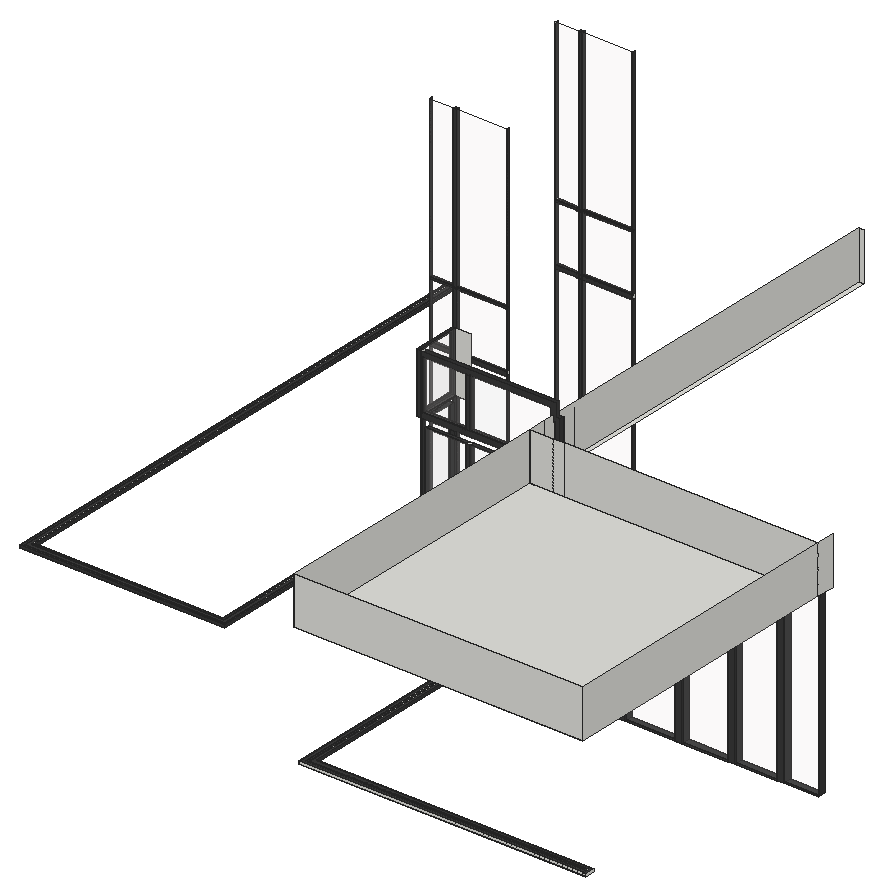
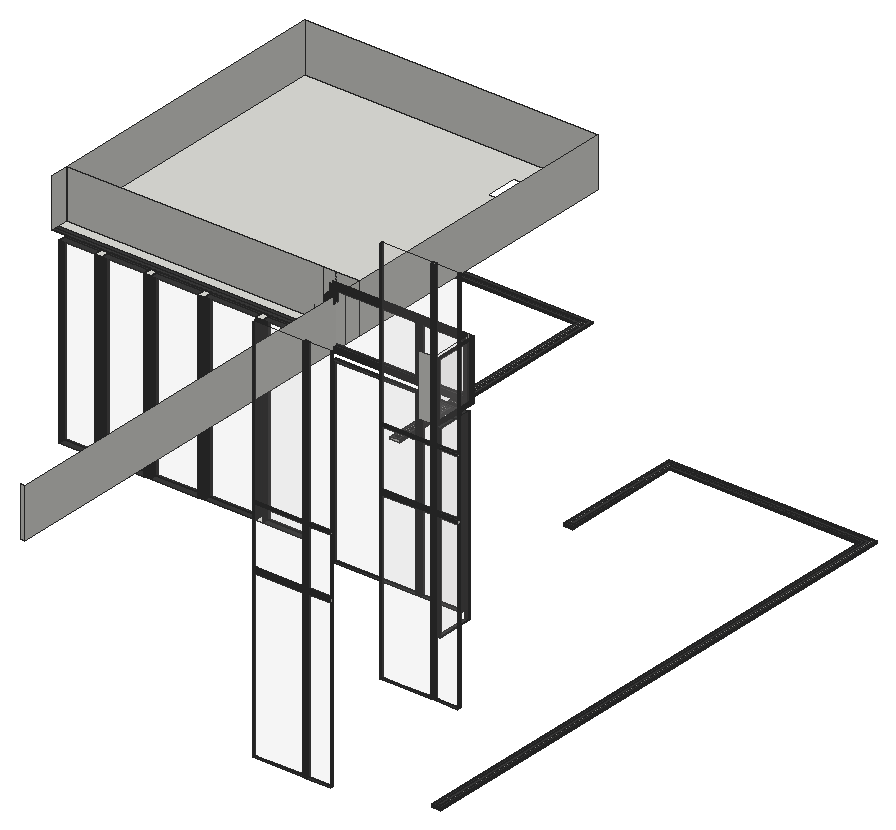
# SketchUp Ruby script. Lengths in inches.
U = 1.inch
M = Sketchup.active_model
def pt(a) = Geom::Point3d.new(a.map { |v| v * U })
def face(e, loops, mat)
  f = e.add_face(loops[0].map { |a| pt(a) })
  loops[1..].each { |l| e.add_face(l.map { |a| pt(a) }).erase! }
  f.material = f.back_material = mat if mat
  f
end
# faces: each face lists its corners as indices into pts; further lists are holes
def faces(e, pts, list, mat = nil) = list.each { |f| face(e, (f[0].is_a?(Array) ? f : [f]).map { |l| l.map { |i| pts[i] } }, mat) }
# xy, xz, yz: faces in a plane at the given z, y or x. An outline is a flat list of corners, or four numbers for a rectangle; further outlines are holes
def ring(l) = l.size == 4 ? [[l[0], l[1]], [l[2], l[1]], [l[2], l[3]], [l[0], l[3]]] : l.each_slice(2).to_a
def flat(e, list, mat, &to3) = list.each { |f| face(e, (f[0].is_a?(Array) ? f : [f]).map { |l| ring(l).map { |u, v| to3.(u, v) } }, mat) }
def xy(e, z, list, mat = nil) = flat(e, list, mat) { |x, y| [x, y, z] }
def xz(e, y, list, mat = nil) = flat(e, list, mat) { |x, z| [x, y, z] }
def yz(e, x, list, mat = nil) = flat(e, list, mat) { |y, z| [x, y, z] }
def lines(e, pts, list) = list.each { |a, b| e.add_line(pt(pts[a]), pt(pts[b])) }
# prism: a flat outline (further loops are holes) pulled along v
def prism(e, loops, v, mat = nil)
  f = face(e, loops, mat); d = Geom::Vector3d.new(v.map { |x| x * U })
  f.pushpull(f.normal.samedirection?(d) ? d.length : -d.length)
end
def box(e, o, s, mat = nil) = prism(e, [[o, [o[0] + s[0], o[1], o[2]], [o[0] + s[0], o[1] + s[1], o[2]], [o[0], o[1] + s[1], o[2]]]], [0, 0, s[2]], mat)
def at(x, y, z, deg = 0) = Geom::Transformation.translation(pt([x, y, z])) * Geom::Transformation.rotation(ORIGIN, Z_AXIS, deg.degrees)
def axes(o, x, y, z) = Geom::Transformation.new([*x, 0, *y, 0, *z, 0, *pt(o).to_a, 1])
def part(name) = M.definitions.add(name)
# library, detail: a bought-in or finely detailed component or shape, given as its bounding box
def library(name, o, s) = part(name).tap { |d| box(d.entities, o, s) }
def detail(e, o, s) = box(e.add_group.entities, o, s)
def put(e, d, t, mat = nil) = e.add_instance(d, t).tap { |i| i.material = mat if mat }
def group(e, t, mat = nil) = e.add_group.tap { |g| g.transformation = t; g.material = mat if mat }.entities
root = M.entities
M.materials.add("Glass Thin Clear 001").color = [255, 250, 250]
M.materials["Glass Thin Clear 001"].alpha = 0.1
M.materials.add("[Color M07]").color = [58, 58, 58]
xy(root,128.05,[[142,272.42,142.4375,280.43],[142.4375,272.42,144.125,280.43],[142,280.43,142.4375,290.07],[142.4375,280.43,144.125,290.07]],"[Color M07]")
xy(root,129.38,[[249.96,260.1875,253.4,264.4375],[278.34,260.1875,281.78,264.4375],[304.65,260.1875,308.09,264.4375],[328.85,260.1875,332.29,264.4375]])
xy(root,129.38,[[230.23,260.1875,249.96,261.1875],[253.4,260.1875,278.34,261.1875],[281.78,260.1875,304.65,261.1875],[308.09,260.1875,328.85,261.1875],[332.29,260.1875,349.62,261.1875],
  [230.23,261.1875,249.96,264.4375],[253.4,261.1875,278.34,264.4375],[281.78,261.1875,304.65,264.4375],[308.09,261.1875,328.85,264.4375],[332.29,261.1875,349.62,264.4375]],"[Color M07]")
xy(root,129.6875,[[166.4375,269.93,168.4375,272.05]])
xy(root,129.6875,[[146.125,269.93,166.4375,270.37],[168.4375,269.93,209.625,270.37],[146.125,270.37,166.4375,272.05],[168.4375,270.37,209.625,272.05]],"[Color M07]")
xy(root,130.31,[[110.9,331.125,112.77,331.5625],[110.9,331.5625,112.77,332.75],[110.9,409.3125,112.77,409.75],[110.9,409.75,112.77,410.9375]])
xy(root,130.31,[[99.31,331.125,110.9,331.5625],[112.77,331.125,131,331.5625],[131,331.125,137.69,331.5625],[99.31,331.5625,110.9,332.75],[112.77,331.5625,131,332.75],
  [131,331.5625,137.69,332.75],[99.31,409.3125,110.9,409.75],[112.77,409.3125,131,409.75],[131,409.3125,137.69,409.75],[99.31,409.75,110.9,410.9375],
  [112.77,409.75,131,410.9375],[131,409.75,137.69,410.9375]],"[Color M07]")
xy(root,162,[[213.57,111.13,213.57,226.42,214.91,226.42,214.91,112.47,353,112.47,353,111.13],[21.25,176.82,21.25,441.31,23.16,441.31,23.16,178.72,118.84,178.72,118.84,238.125,120.75,238.125,120.75,176.82]])
xy(root,162,[[[211.8125,109.375,211.8125,228.18,216.67,228.18,216.67,114.23,354.76,114.23,354.76,109.375],[213.57,111.13,353,111.13,353,112.47,214.91,112.47,214.91,226.42,213.57,226.42]],[[20,175.57,20,442.56,24.41,442.56,24.41,179.97,117.59,179.97,117.59,239.37,122,239.37,122,175.57],[21.25,176.82,120.75,176.82,120.75,238.125,118.84,238.125,118.84,178.72,23.16,178.72,23.16,441.31,21.25,441.31]]],"[Color M07]")
xy(root,163.1875,[[[211.8125,109.375,354.76,109.375,354.76,114.23,216.67,114.23,216.67,228.18,211.8125,228.18],[213.57,111.13,213.57,226.42,214.91,226.42,214.91,112.47,353,112.47,353,111.13]],[213.57,111.13,353,111.13,353,112.47,214.91,112.47,214.91,226.42,213.57,226.42],[[20,175.57,122,175.57,122,239.37,117.59,239.37,117.59,179.97,24.41,179.97,24.41,442.56,20,442.56],[21.25,176.82,21.25,441.31,23.16,441.31,23.16,178.72,118.84,178.72,118.84,238.125,120.75,238.125,120.75,176.82]],[21.25,176.82,120.75,176.82,120.75,238.125,118.84,238.125,118.84,178.72,23.16,178.72,23.16,441.31,21.25,441.31]],"[Color M07]")
xy(root,211.33,[[110.9,331.125,112.77,331.5625],[110.9,331.5625,112.77,332.75],[110.9,409.3125,112.77,409.75],[110.9,409.75,112.77,410.9375]])
xy(root,211.33,[[99.31,331.125,110.9,331.5625],[112.77,331.125,137.69,331.5625],[99.31,331.5625,110.9,332.75],[112.77,331.5625,137.69,332.75],[99.31,409.3125,110.9,409.75],
  [112.77,409.3125,137.69,409.75],[99.31,409.75,110.9,410.9375],[112.77,409.75,137.69,410.9375]],"[Color M07]")
xy(root,213.22,[[110.9,331.125,112.77,331.5625],[110.9,331.5625,112.77,332.75],[110.9,409.3125,112.77,409.75],[110.9,409.75,112.77,410.9375]])
xy(root,213.22,[[99.31,331.125,110.9,331.5625],[112.77,331.125,137.69,331.5625],[99.31,331.5625,110.9,332.75],[112.77,331.5625,137.69,332.75],[99.31,409.3125,110.9,409.75],
  [112.77,409.3125,137.69,409.75],[99.31,409.75,110.9,410.9375],[112.77,409.75,137.69,410.9375]],"[Color M07]")
xy(root,218.3125,[[166.4375,269.93,168.4375,272.05]])
xy(root,218.3125,[[146.125,269.93,166.4375,270.37],[168.4375,269.93,209.625,270.37],[146.125,270.37,166.4375,272.05],[168.4375,270.37,209.625,272.05]],"[Color M07]")
xy(root,218.62,[[249.96,260.1875,253.4,264.4375],[278.34,260.1875,281.78,264.4375],[304.65,260.1875,308.09,264.4375],[328.85,260.1875,332.29,264.4375]])
xy(root,218.62,[[230.23,260.1875,249.96,261.1875],[253.4,260.1875,278.34,261.1875],[281.78,260.1875,304.65,261.1875],[308.09,260.1875,328.85,261.1875],[332.29,260.1875,349.62,261.1875],
  [230.23,261.1875,249.96,264.4375],[253.4,261.1875,278.34,264.4375],[281.78,261.1875,304.65,264.4375],[308.09,261.1875,328.85,264.4375],[332.29,261.1875,349.62,264.4375]],"[Color M07]")
xy(root,219.95,[[142,272.42,142.4375,280.43],[142.4375,272.42,144.125,280.43],[142,280.43,142.4375,290.07],[142.4375,280.43,144.125,290.07]],"[Color M07]")
xy(root,222,[[[209.4375,109.375,353,255.6875],[220.8125,122.73,239.9375,139.05]],[209.4375,255.6875,211.8125,264.6875],[226.85,255.6875,353,260.1875],[226.85,264.4375,353,264.6875],[209.4375,264.6875,211.8125,269.93],
  [210.9375,269.93,211.8125,271.43],[211.8125,269.93,213.3125,271.43],[210.9375,271.43,211.8125,272.05],[211.8125,271.43,213.3125,272.05],[209.4375,272.05,211.8125,280.43],
  [209.4375,280.43,211.8125,460.5625]])
xy(root,222,[[226.85,260.1875,353,262.625],[226.85,262.625,353,264.4375],[142,269.93,143.5,271.43],[143.5,269.93,144.125,271.43],[144.125,269.93,209.4375,271.43],
  [209.4375,269.93,210.9375,271.43],[142,271.43,143.5,272.05],[143.5,271.43,144.125,272.05],[144.125,271.43,209.4375,272.05],[209.4375,271.43,210.9375,272.05],
  [142,272.05,143.5,280.43],[143.5,272.05,144.125,280.43],[142,280.43,143.5,292.12],[143.5,280.43,144.125,292.12]],"[Color M07]")
xy(root,223.64,[[142,272.01,142.4375,272.05],[142.4375,272.01,144.125,272.05],[142,272.05,142.4375,290.47]])
xy(root,224.5,[[166.4375,269.93,168.4375,272.05]])
xy(root,224.5,[[144.9375,269.93,166.4375,270.37],[168.4375,269.93,210.8125,270.37],[144.9375,270.37,166.4375,272.05],[168.4375,270.37,210.8125,272.05]],"[Color M07]")
xy(root,241.3125,[[110.9,331.125,112.77,331.5625],[110.9,331.5625,112.77,332.75],[110.9,409.3125,112.77,409.75],[110.9,409.75,112.77,410.9375]])
xy(root,241.3125,[[99.31,331.125,110.9,331.5625],[112.77,331.125,137.69,331.5625],[99.31,331.5625,110.9,332.75],[112.77,331.5625,137.69,332.75],[99.31,409.3125,110.9,409.75],
  [112.77,409.3125,137.69,409.75],[99.31,409.75,110.9,410.9375],[112.77,409.75,137.69,410.9375]],"[Color M07]")
xy(root,242.24,[[110.9,331.125,112.77,331.5625],[110.9,331.5625,112.77,332.75],[110.9,409.3125,112.77,409.75],[110.9,409.75,112.77,410.9375]])
xy(root,242.24,[[99.31,331.125,110.9,331.5625],[112.77,331.125,137.69,331.5625],[99.31,331.5625,110.9,332.75],[112.77,331.5625,137.69,332.75],[99.31,409.3125,110.9,409.75],
  [112.77,409.3125,137.69,409.75],[99.31,409.75,110.9,410.9375],[112.77,409.75,137.69,410.9375]],"[Color M07]")
xz(root,109.375,[[211.8125,162,353,163.1875],[353,162,354.76,163.1875],[209.4375,222,353,246]])
xz(root,111.13,[[213.57,162,353,163.1875]])
xz(root,112.47,[[214.91,162,353,163.1875]])
xz(root,114.23,[[216.67,162,354.76,163.1875]],"[Color M07]")
xz(root,175.57,[[20,162,122,163.1875]],"[Color M07]")
xz(root,176.82,[[21.25,162,120.75,163.1875]])
xz(root,178.72,[[23.16,162,118.84,163.1875]])
xz(root,179.97,[[24.41,162,117.59,163.1875]],"[Color M07]")
xz(root,226.42,[[213.57,162,214.91,163.1875]])
xz(root,228.18,[[211.8125,162,216.67,163.1875]])
xz(root,238.125,[[118.84,162,120.75,163.1875]])
xz(root,239.37,[[117.59,162,122,163.1875]],"[Color M07]")
xz(root,255.6875,[[209.4375,222,220.8125,246],[220.8125,222,226.85,246],[226.85,222,353,246]])
xz(root,260.1875,[[249.96,129.38,253.4,218.62],[278.34,129.38,281.78,218.62],[304.65,129.38,308.09,218.62],[328.85,129.38,332.29,218.62]],"[Color M07]")
xz(root,261.1875,[[230.23,129.38,249.96,218.62],[253.4,129.38,278.34,218.62],[281.78,129.38,304.65,218.62],[308.09,129.38,328.85,218.62],[332.29,129.38,349.62,218.62]],"Glass Thin Clear 001")
xz(root,264.4375,[[278.34,129.38,281.78,218.62],[304.65,129.38,308.09,218.62],[328.85,129.38,332.29,218.62]],"[Color M07]")
xz(root,269.93,[[166.4375,129.6875,168.4375,218.3125],[142,222,144.125,252],[[144.125,222,213.3125,222,213.3125,246,210.9375,246,210.9375,252,144.125,252],[144.9375,224.5,144.9375,249.5,208.4375,249.5,208.4375,243.5,210.8125,243.5,210.8125,224.5]],[166.4375,224.5,168.4375,249.5]],"[Color M07]")
xz(root,270.37,[[146.125,129.6875,166.4375,218.3125],[168.4375,129.6875,209.625,218.3125],[144.9375,224.5,166.4375,249.5],[168.4375,224.5,210.8125,224.5,210.8125,243.5,208.4375,243.5,208.4375,249.5,168.4375,249.5]],"Glass Thin Clear 001")
xz(root,272.01,[[142,223.64,142.4375,250.36],[142.4375,223.64,144.125,250.36]])
xz(root,272.05,[[166.4375,129.6875,168.4375,218.3125],[142,222,144.125,223.64],[[144.125,222,144.125,223.64,142,223.64,142,250.36,144.125,250.36,144.125,252,210.9375,252,210.9375,246,213.3125,246,213.3125,222],[144.9375,224.5,210.8125,224.5,210.8125,243.5,208.4375,243.5,208.4375,249.5,144.9375,249.5]],[166.4375,224.5,168.4375,249.5]],"[Color M07]")
xz(root,272.42,[[142,128.05,142.4375,219.95],[142.4375,128.05,144.125,219.95]],"[Color M07]")
xz(root,290.07,[[142,128.05,142.4375,219.95],[142.4375,128.05,144.125,219.95]],"[Color M07]")
xz(root,290.47,[[142,223.64,142.4375,250.36]],"[Color M07]")
xz(root,292.12,[[143.5,222,151,252]])
xz(root,292.12,[[142,222,143.5,252]],"[Color M07]")
xz(root,331.125,[[110.9,130.31,112.77,211.33],[99.31,211.33,110.9,213.22],[110.9,211.33,112.77,213.22],[112.77,211.33,137.69,213.22],[110.9,213.22,112.77,241.3125],
  [99.31,241.3125,110.9,242.24],[110.9,241.3125,112.77,242.24],[112.77,241.3125,137.69,242.24],[110.9,242.24,112.77,321.57]],"[Color M07]")
xz(root,331.5625,[[110.9,130.31,112.77,211.33],[99.31,211.33,110.9,213.22],[110.9,211.33,112.77,213.22],[112.77,211.33,137.69,213.22],[110.9,213.22,112.77,241.3125],
  [99.31,241.3125,110.9,242.24],[110.9,241.3125,112.77,242.24],[112.77,241.3125,137.69,242.24],[110.9,242.24,112.77,321.57]])
xz(root,331.5625,[[99.31,130.31,110.9,211.33],[112.77,130.31,137.69,211.33],[99.31,213.22,110.9,241.3125],[112.77,213.22,137.69,241.3125],[99.31,242.24,110.9,321.57],
  [112.77,242.24,137.69,321.57]],"Glass Thin Clear 001")
xz(root,332.75,[[110.9,130.31,112.77,211.33],[99.31,211.33,110.9,213.22],[110.9,211.33,112.77,213.22],[112.77,211.33,137.69,213.22],[110.9,213.22,112.77,241.3125],
  [99.31,241.3125,110.9,242.24],[110.9,241.3125,112.77,242.24],[112.77,241.3125,137.69,242.24],[110.9,242.24,112.77,321.57]],"[Color M07]")
xz(root,409.3125,[[110.9,130.31,112.77,211.33],[99.31,211.33,110.9,213.22],[110.9,211.33,112.77,213.22],[112.77,211.33,137.69,213.22],[110.9,213.22,112.77,241.3125],
  [99.31,241.3125,110.9,242.24],[110.9,241.3125,112.77,242.24],[112.77,241.3125,137.69,242.24],[110.9,242.24,112.77,321.57]],"[Color M07]")
xz(root,409.75,[[110.9,130.31,112.77,211.33],[99.31,211.33,110.9,213.22],[110.9,211.33,112.77,213.22],[112.77,211.33,137.69,213.22],[110.9,213.22,112.77,241.3125],
  [99.31,241.3125,110.9,242.24],[110.9,241.3125,112.77,242.24],[112.77,241.3125,137.69,242.24],[110.9,242.24,112.77,321.57]])
xz(root,409.75,[[99.31,130.31,110.9,211.33],[112.77,130.31,137.69,211.33],[99.31,213.22,110.9,241.3125],[112.77,213.22,137.69,241.3125],[99.31,242.24,110.9,321.57],
  [112.77,242.24,137.69,321.57]],"Glass Thin Clear 001")
xz(root,410.9375,[[110.9,130.31,112.77,211.33],[99.31,211.33,110.9,213.22],[110.9,211.33,112.77,213.22],[112.77,211.33,137.69,213.22],[110.9,213.22,112.77,241.3125],
  [99.31,241.3125,110.9,242.24],[110.9,241.3125,112.77,242.24],[112.77,241.3125,137.69,242.24],[110.9,242.24,112.77,321.57]],"[Color M07]")
xz(root,441.31,[[21.25,162,23.16,163.1875]])
xz(root,442.56,[[20,162,24.41,163.1875]],"[Color M07]")
xz(root,460.5625,[[209.4375,222,211.8125,246]])
yz(root,20,[[175.57,162,442.56,163.1875]],"[Color M07]")
yz(root,21.25,[[176.82,162,441.31,163.1875]])
yz(root,23.16,[[178.72,162,441.31,163.1875]])
yz(root,24.41,[[179.97,162,442.56,163.1875]],"[Color M07]")
yz(root,99.31,[[331.125,130.31,331.5625,211.33],[409.3125,130.31,409.75,211.33],[331.125,211.33,331.5625,213.22],[331.5625,211.33,332.75,213.22],[409.3125,211.33,409.75,213.22],
  [409.75,211.33,410.9375,213.22],[331.125,241.3125,331.5625,242.24],[331.5625,241.3125,332.75,242.24],[409.3125,241.3125,409.75,242.24],[409.75,241.3125,410.9375,242.24],
  [331.125,242.24,331.5625,321.57],[409.3125,242.24,409.75,321.57]])
yz(root,99.31,[[331.5625,130.31,332.75,211.33],[409.75,130.31,410.9375,211.33],[331.125,213.22,331.5625,241.3125],[331.5625,213.22,332.75,241.3125],[409.3125,213.22,409.75,241.3125],
  [409.75,213.22,410.9375,241.3125],[331.5625,242.24,332.75,321.57],[409.75,242.24,410.9375,321.57]],"[Color M07]")
yz(root,110.9,[[331.125,211.33,331.5625,213.22],[331.5625,211.33,332.75,213.22],[409.3125,211.33,409.75,213.22],[409.75,211.33,410.9375,213.22],[331.125,241.3125,331.5625,242.24],
  [331.5625,241.3125,332.75,242.24],[409.3125,241.3125,409.75,242.24],[409.75,241.3125,410.9375,242.24]])
yz(root,110.9,[[331.125,130.31,331.5625,211.33],[331.5625,130.31,332.75,211.33],[409.3125,130.31,409.75,211.33],[409.75,130.31,410.9375,211.33],[331.125,213.22,331.5625,241.3125],
  [331.5625,213.22,332.75,241.3125],[409.3125,213.22,409.75,241.3125],[409.75,213.22,410.9375,241.3125],[331.125,242.24,331.5625,321.57],[331.5625,242.24,332.75,321.57],
  [409.3125,242.24,409.75,321.57],[409.75,242.24,410.9375,321.57]],"[Color M07]")
yz(root,112.77,[[331.125,130.31,331.5625,211.33],[409.3125,130.31,409.75,211.33],[331.125,211.33,331.5625,213.22],[331.5625,211.33,332.75,213.22],[409.3125,211.33,409.75,213.22],
  [409.75,211.33,410.9375,213.22],[331.125,241.3125,331.5625,242.24],[331.5625,241.3125,332.75,242.24],[409.3125,241.3125,409.75,242.24],[409.75,241.3125,410.9375,242.24]])
yz(root,112.77,[[331.5625,130.31,332.75,211.33],[409.75,130.31,410.9375,211.33],[331.125,213.22,331.5625,241.3125],[331.5625,213.22,332.75,241.3125],[409.3125,213.22,409.75,241.3125],
  [409.75,213.22,410.9375,241.3125],[331.125,242.24,331.5625,321.57],[331.5625,242.24,332.75,321.57],[409.3125,242.24,409.75,321.57],[409.75,242.24,410.9375,321.57]],"[Color M07]")
yz(root,117.59,[[179.97,162,239.37,163.1875]],"[Color M07]")
yz(root,118.84,[[178.72,162,238.125,163.1875]])
yz(root,120.75,[[176.82,162,238.125,163.1875]])
yz(root,122,[[175.57,162,239.37,163.1875]],"[Color M07]")
yz(root,137.69,[[331.125,211.33,331.5625,213.22],[331.5625,211.33,332.75,213.22],[409.3125,211.33,409.75,213.22],[409.75,211.33,410.9375,213.22],[331.125,241.3125,331.5625,242.24],
  [331.5625,241.3125,332.75,242.24],[409.3125,241.3125,409.75,242.24],[409.75,241.3125,410.9375,242.24]])
yz(root,137.69,[[331.125,130.31,331.5625,211.33],[331.5625,130.31,332.75,211.33],[409.3125,130.31,409.75,211.33],[409.75,130.31,410.9375,211.33],[331.125,213.22,331.5625,241.3125],
  [331.5625,213.22,332.75,241.3125],[409.3125,213.22,409.75,241.3125],[409.75,213.22,410.9375,241.3125],[331.125,242.24,331.5625,321.57],[331.5625,242.24,332.75,321.57],
  [409.3125,242.24,409.75,321.57],[409.75,242.24,410.9375,321.57]],"[Color M07]")
yz(root,142,[[272.01,223.64,272.05,250.36]])
yz(root,142,[[269.93,222,269.93,252,272.05,252,272.05,250.36,272.01,250.36,272.01,223.64,272.05,223.64,272.05,222],[272.05,222,272.05,223.64,290.47,223.64,290.47,250.36,272.05,250.36,272.05,252,292.12,252,292.12,222]],"[Color M07]")
yz(root,142.4375,[[272.42,128.05,290.07,219.95],[272.01,223.64,290.47,250.36]],"Glass Thin Clear 001")
yz(root,143.5,[[271.43,222,292.12,252]],"Glass Thin Clear 001")
yz(root,144.125,[[269.93,222,272.05,222,272.05,223.64,272.01,223.64,272.01,250.36,272.05,250.36,272.05,252,269.93,252]])
yz(root,144.9375,[[269.93,224.5,270.37,249.5],[270.37,224.5,272.05,249.5]],"[Color M07]")
yz(root,146.125,[[269.93,129.6875,270.37,218.3125],[270.37,129.6875,272.05,218.3125]],"[Color M07]")
yz(root,166.4375,[[269.93,129.6875,270.37,218.3125],[270.37,129.6875,272.05,218.3125],[269.93,224.5,270.37,249.5],[270.37,224.5,272.05,249.5]],"[Color M07]")
yz(root,168.4375,[[269.93,129.6875,270.37,218.3125],[270.37,129.6875,272.05,218.3125],[269.93,224.5,270.37,249.5],[270.37,224.5,272.05,249.5]],"[Color M07]")
yz(root,209.4375,[[109.375,222,255.6875,246],[255.6875,222,264.6875,246],[264.6875,222,460.5625,246]])
yz(root,209.625,[[269.93,129.6875,270.37,218.3125],[270.37,129.6875,272.05,218.3125]],"[Color M07]")
yz(root,210.8125,[[269.93,224.5,270.37,243.5],[270.37,224.5,272.05,243.5]],"[Color M07]")
yz(root,211.8125,[[109.375,162,228.18,163.1875]],"[Color M07]")
yz(root,213.3125,[[269.93,222,271.43,246],[271.43,222,272.05,246]],"[Color M07]")
yz(root,213.57,[[111.13,162,226.42,163.1875]])
yz(root,214.91,[[112.47,162,226.42,163.1875]])
yz(root,216.67,[[114.23,162,228.18,163.1875]],"[Color M07]")
yz(root,230.23,[[260.1875,129.38,261.1875,218.62],[261.1875,129.38,264.4375,218.62]],"[Color M07]")
yz(root,249.96,[[260.1875,129.38,261.1875,218.62],[261.1875,129.38,264.4375,218.62]],"[Color M07]")
yz(root,253.4,[[260.1875,129.38,261.1875,218.62],[261.1875,129.38,264.4375,218.62]],"[Color M07]")
yz(root,278.34,[[260.1875,129.38,261.1875,218.62],[261.1875,129.38,264.4375,218.62]],"[Color M07]")
yz(root,281.78,[[260.1875,129.38,261.1875,218.62],[261.1875,129.38,264.4375,218.62]],"[Color M07]")
yz(root,304.65,[[260.1875,129.38,261.1875,218.62],[261.1875,129.38,264.4375,218.62]],"[Color M07]")
yz(root,308.09,[[260.1875,129.38,261.1875,218.62],[261.1875,129.38,264.4375,218.62]],"[Color M07]")
yz(root,328.85,[[260.1875,129.38,261.1875,218.62],[261.1875,129.38,264.4375,218.62]],"[Color M07]")
yz(root,332.29,[[260.1875,129.38,261.1875,218.62],[261.1875,129.38,264.4375,218.62]],"[Color M07]")
yz(root,349.62,[[260.1875,129.38,261.1875,218.62],[261.1875,129.38,264.4375,218.62]],"[Color M07]")
yz(root,353,[[111.13,162,112.47,163.1875],[109.375,222,255.6875,246],[255.6875,222,264.6875,246]])
yz(root,354.76,[[109.375,162,114.23,163.1875]])
p = [[211.8125,280.43,222],[211.8125,280.43,246]]
lines(root,p,[[0,1]])
